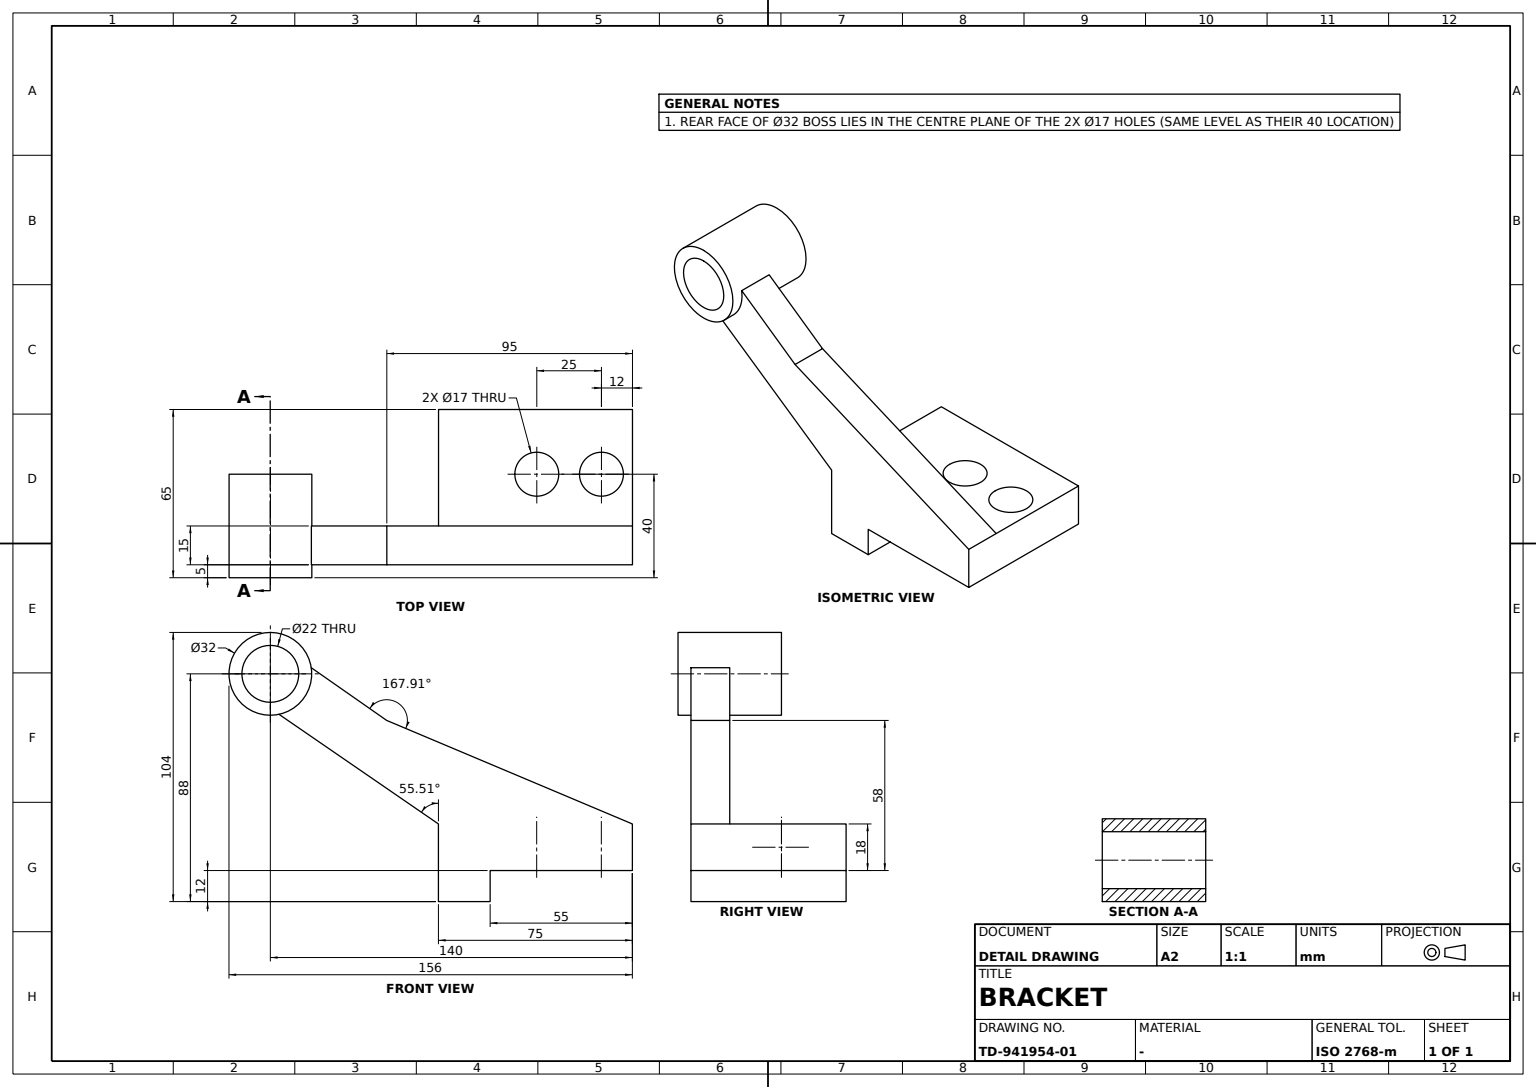
ISO-10303-21;
HEADER;
FILE_DESCRIPTION((''),'2;1');
FILE_NAME('','',(''),(''),'','','');
FILE_SCHEMA(('AUTOMOTIVE_DESIGN'));
ENDSEC;
DATA;
#1=APPLICATION_CONTEXT('');
#2=PRODUCT_CONTEXT('',#1,'mechanical');
#3=PRODUCT('','','',(#2));
#4=PRODUCT_DEFINITION_FORMATION('','',#3);
#5=PRODUCT_DEFINITION_CONTEXT('',#1,'design');
#6=PRODUCT_DEFINITION('','',#4,#5);
#7=PRODUCT_DEFINITION_SHAPE('','',#6);
#8=(LENGTH_UNIT()NAMED_UNIT(*)SI_UNIT(.MILLI.,.METRE.));
#9=(NAMED_UNIT(*)PLANE_ANGLE_UNIT()SI_UNIT($,.RADIAN.));
#10=(NAMED_UNIT(*)SI_UNIT($,.STERADIAN.)SOLID_ANGLE_UNIT());
#11=UNCERTAINTY_MEASURE_WITH_UNIT(LENGTH_MEASURE(0.005),#8,'distance_accuracy_value','');
#12=(GEOMETRIC_REPRESENTATION_CONTEXT(3)GLOBAL_UNCERTAINTY_ASSIGNED_CONTEXT((#11))GLOBAL_UNIT_ASSIGNED_CONTEXT((#8,#9,#10))REPRESENTATION_CONTEXT('',''));
#13=CARTESIAN_POINT('',(-140.,35.,92.));
#14=VERTEX_POINT('',#13);
#15=CARTESIAN_POINT('',(-140.,35.,76.));
#16=DIRECTION('',(0.,1.,0.));
#17=DIRECTION('',(0.,0.,1.));
#18=AXIS2_PLACEMENT_3D('',#15,#16,#17);
#19=CIRCLE('',#18,16.);
#20=EDGE_CURVE('',#14,#14,#19,.T.);
#21=ORIENTED_EDGE('',*,*,#20,.T.);
#22=EDGE_LOOP('',(#21));
#23=FACE_BOUND('',#22,.T.);
#24=CARTESIAN_POINT('',(-140.,35.,87.));
#25=VERTEX_POINT('',#24);
#26=CIRCLE('',#18,11.);
#27=EDGE_CURVE('',#25,#25,#26,.T.);
#28=ORIENTED_EDGE('',*,*,#27,.F.);
#29=EDGE_LOOP('',(#28));
#30=FACE_BOUND('',#29,.T.);
#31=CARTESIAN_POINT('',(0.,35.,0.));
#32=DIRECTION('',(-1.,0.,0.));
#33=AXIS2_PLACEMENT_3D('',#31,#16,#32);
#34=PLANE('',#33);
#35=ADVANCED_FACE('',(#23,#30),#34,.T.);
#36=CARTESIAN_POINT('',(-3.5,35.,0.));
#37=VERTEX_POINT('',#36);
#38=CARTESIAN_POINT('',(-12.,35.,0.));
#39=DIRECTION('',(1.,0.,0.));
#40=AXIS2_PLACEMENT_3D('',#38,#17,#39);
#41=CIRCLE('',#40,8.5);
#42=EDGE_CURVE('',#37,#37,#41,.T.);
#43=ORIENTED_EDGE('',*,*,#42,.F.);
#44=EDGE_LOOP('',(#43));
#45=FACE_BOUND('',#44,.T.);
#46=CARTESIAN_POINT('',(-20.5,35.,18.));
#47=VERTEX_POINT('',#46);
#48=CARTESIAN_POINT('',(-12.,35.,18.));
#49=DIRECTION('',(0.,0.,-1.));
#50=AXIS2_PLACEMENT_3D('',#48,#49,#32);
#51=CIRCLE('',#50,8.5);
#52=EDGE_CURVE('',#47,#47,#51,.T.);
#53=ORIENTED_EDGE('',*,*,#52,.F.);
#54=EDGE_LOOP('',(#53));
#55=FACE_BOUND('',#54,.T.);
#56=CARTESIAN_POINT('',(-12.,35.,10.));
#57=AXIS2_PLACEMENT_3D('',#56,#17,#39);
#58=CYLINDRICAL_SURFACE('',#57,8.5);
#59=ADVANCED_FACE('',(#45,#55),#58,.F.);
#60=CARTESIAN_POINT('',(-124.176279,0.,78.368516));
#61=VERTEX_POINT('',#60);
#62=CARTESIAN_POINT('',(-136.651894,0.,60.354228));
#63=VERTEX_POINT('',#62);
#64=CARTESIAN_POINT('',(-140.,0.,76.));
#65=AXIS2_PLACEMENT_3D('',#64,#16,#17);
#66=CIRCLE('',#65,16.);
#67=EDGE_CURVE('',#61,#63,#66,.T.);
#68=ORIENTED_EDGE('',*,*,#67,.T.);
#69=CARTESIAN_POINT('',(-75.,0.,18.));
#70=VERTEX_POINT('',#69);
#71=CARTESIAN_POINT('',(-15.646411,0.,-22.775315));
#72=DIRECTION('',(-0.824238161,0.,0.566243282));
#73=VECTOR('',#72,1000.);
#74=LINE('',#71,#73);
#75=EDGE_CURVE('',#70,#63,#74,.T.);
#76=ORIENTED_EDGE('',*,*,#75,.F.);
#77=CARTESIAN_POINT('',(-75.,0.,-12.));
#78=VERTEX_POINT('',#77);
#79=CARTESIAN_POINT('',(-75.,0.,0.));
#80=VECTOR('',#49,1000.);
#81=LINE('',#79,#80);
#82=EDGE_CURVE('',#70,#78,#81,.T.);
#83=ORIENTED_EDGE('',*,*,#82,.T.);
#84=CARTESIAN_POINT('',(-55.,0.,-12.));
#85=VERTEX_POINT('',#84);
#86=CARTESIAN_POINT('',(0.,0.,-12.));
#87=VECTOR('',#39,1000.);
#88=LINE('',#86,#87);
#89=EDGE_CURVE('',#78,#85,#88,.T.);
#90=ORIENTED_EDGE('',*,*,#89,.T.);
#91=CARTESIAN_POINT('',(-55.,0.,0.));
#92=VERTEX_POINT('',#91);
#93=VECTOR('',#17,1000.);
#94=LINE('',#91,#93);
#95=EDGE_CURVE('',#85,#92,#94,.T.);
#96=ORIENTED_EDGE('',*,*,#95,.T.);
#97=CARTESIAN_POINT('',(0.,0.,0.));
#98=VERTEX_POINT('',#97);
#99=LINE('',#97,#87);
#100=EDGE_CURVE('',#92,#98,#99,.T.);
#101=ORIENTED_EDGE('',*,*,#100,.T.);
#102=CARTESIAN_POINT('',(0.,0.,18.));
#103=VERTEX_POINT('',#102);
#104=LINE('',#97,#93);
#105=EDGE_CURVE('',#98,#103,#104,.T.);
#106=ORIENTED_EDGE('',*,*,#105,.T.);
#107=CARTESIAN_POINT('',(-95.,0.,58.));
#108=VERTEX_POINT('',#107);
#109=CARTESIAN_POINT('',(6.437647,0.,15.289412));
#110=DIRECTION('',(-0.921635375,0.,0.388057));
#111=VECTOR('',#110,1000.);
#112=LINE('',#109,#111);
#113=EDGE_CURVE('',#103,#108,#112,.T.);
#114=ORIENTED_EDGE('',*,*,#113,.T.);
#115=CARTESIAN_POINT('',(-3.905728,0.,-5.594645));
#116=DIRECTION('',(-0.819955841,0.,0.572426781));
#117=VECTOR('',#116,1000.);
#118=LINE('',#115,#117);
#119=EDGE_CURVE('',#108,#61,#118,.T.);
#120=ORIENTED_EDGE('',*,*,#119,.T.);
#121=EDGE_LOOP('',(#68,#76,#83,#90,#96,#101,#106,#114,#120));
#122=FACE_BOUND('',#121,.T.);
#123=AXIS2_PLACEMENT_3D('',#97,#16,#32);
#124=PLANE('',#123);
#125=ADVANCED_FACE('',(#122),#124,.F.);
#126=CARTESIAN_POINT('',(-140.,-5.,87.));
#127=VERTEX_POINT('',#126);
#128=CARTESIAN_POINT('',(-140.,-5.,76.));
#129=AXIS2_PLACEMENT_3D('',#128,#16,#17);
#130=CIRCLE('',#129,11.);
#131=EDGE_CURVE('',#127,#127,#130,.T.);
#132=ORIENTED_EDGE('',*,*,#131,.F.);
#133=EDGE_LOOP('',(#132));
#134=FACE_BOUND('',#133,.T.);
#135=ORIENTED_EDGE('',*,*,#27,.T.);
#136=EDGE_LOOP('',(#135));
#137=FACE_BOUND('',#136,.T.);
#138=CARTESIAN_POINT('',(-140.,-2.5,76.));
#139=AXIS2_PLACEMENT_3D('',#138,#16,#32);
#140=CYLINDRICAL_SURFACE('',#139,11.);
#141=ADVANCED_FACE('',(#134,#137),#140,.F.);
#142=ORIENTED_EDGE('',*,*,#75,.T.);
#143=CARTESIAN_POINT('',(-136.651894,15.,60.354228));
#144=VERTEX_POINT('',#143);
#145=VECTOR('',#16,1000.);
#146=LINE('',#62,#145);
#147=EDGE_CURVE('',#63,#144,#146,.T.);
#148=ORIENTED_EDGE('',*,*,#147,.T.);
#149=CARTESIAN_POINT('',(-75.,15.,18.));
#150=VERTEX_POINT('',#149);
#151=CARTESIAN_POINT('',(-15.646411,15.,-22.775315));
#152=LINE('',#151,#73);
#153=EDGE_CURVE('',#150,#144,#152,.T.);
#154=ORIENTED_EDGE('',*,*,#153,.F.);
#155=LINE('',#69,#145);
#156=EDGE_CURVE('',#70,#150,#155,.T.);
#157=ORIENTED_EDGE('',*,*,#156,.F.);
#158=EDGE_LOOP('',(#142,#148,#154,#157));
#159=FACE_BOUND('',#158,.T.);
#160=DIRECTION('',(-0.566243282,0.,-0.824238161));
#161=AXIS2_PLACEMENT_3D('',#69,#160,#72);
#162=PLANE('',#161);
#163=ADVANCED_FACE('',(#159),#162,.T.);
#164=CARTESIAN_POINT('',(-140.,-5.,92.));
#165=VERTEX_POINT('',#164);
#166=CIRCLE('',#129,16.);
#167=EDGE_CURVE('',#165,#165,#166,.T.);
#168=ORIENTED_EDGE('',*,*,#167,.T.);
#169=EDGE_LOOP('',(#168));
#170=FACE_BOUND('',#169,.T.);
#171=ORIENTED_EDGE('',*,*,#20,.F.);
#172=EDGE_LOOP('',(#171));
#173=FACE_BOUND('',#172,.T.);
#174=CARTESIAN_POINT('',(-124.176279,15.,78.368516));
#175=VERTEX_POINT('',#174);
#176=LINE('',#60,#145);
#177=EDGE_CURVE('',#61,#175,#176,.T.);
#178=ORIENTED_EDGE('',*,*,#177,.T.);
#179=CARTESIAN_POINT('',(-140.,15.,76.));
#180=AXIS2_PLACEMENT_3D('',#179,#16,#17);
#181=CIRCLE('',#180,16.);
#182=EDGE_CURVE('',#175,#144,#181,.T.);
#183=ORIENTED_EDGE('',*,*,#182,.T.);
#184=ORIENTED_EDGE('',*,*,#147,.F.);
#185=ORIENTED_EDGE('',*,*,#67,.F.);
#186=EDGE_LOOP('',(#178,#183,#184,#185));
#187=FACE_BOUND('',#186,.T.);
#188=CARTESIAN_POINT('',(-140.,7.5,76.));
#189=AXIS2_PLACEMENT_3D('',#188,#16,#32);
#190=CYLINDRICAL_SURFACE('',#189,16.);
#191=ADVANCED_FACE('',(#170,#173,#187),#190,.T.);
#192=CARTESIAN_POINT('',(-55.,60.,-12.));
#193=VERTEX_POINT('',#192);
#194=LINE('',#84,#145);
#195=EDGE_CURVE('',#85,#193,#194,.T.);
#196=ORIENTED_EDGE('',*,*,#195,.F.);
#197=ORIENTED_EDGE('',*,*,#89,.F.);
#198=CARTESIAN_POINT('',(-75.,60.,-12.));
#199=VERTEX_POINT('',#198);
#200=LINE('',#77,#145);
#201=EDGE_CURVE('',#78,#199,#200,.T.);
#202=ORIENTED_EDGE('',*,*,#201,.T.);
#203=CARTESIAN_POINT('',(0.,60.,-12.));
#204=LINE('',#203,#87);
#205=EDGE_CURVE('',#199,#193,#204,.T.);
#206=ORIENTED_EDGE('',*,*,#205,.T.);
#207=EDGE_LOOP('',(#196,#197,#202,#206));
#208=FACE_BOUND('',#207,.T.);
#209=AXIS2_PLACEMENT_3D('',#77,#17,#39);
#210=PLANE('',#209);
#211=ADVANCED_FACE('',(#208),#210,.F.);
#212=CARTESIAN_POINT('',(0.,15.,18.));
#213=VERTEX_POINT('',#212);
#214=LINE('',#102,#145);
#215=EDGE_CURVE('',#103,#213,#214,.T.);
#216=ORIENTED_EDGE('',*,*,#215,.T.);
#217=CARTESIAN_POINT('',(-95.,15.,58.));
#218=VERTEX_POINT('',#217);
#219=CARTESIAN_POINT('',(6.437647,15.,15.289412));
#220=LINE('',#219,#111);
#221=EDGE_CURVE('',#213,#218,#220,.T.);
#222=ORIENTED_EDGE('',*,*,#221,.T.);
#223=LINE('',#107,#145);
#224=EDGE_CURVE('',#108,#218,#223,.T.);
#225=ORIENTED_EDGE('',*,*,#224,.F.);
#226=ORIENTED_EDGE('',*,*,#113,.F.);
#227=EDGE_LOOP('',(#216,#222,#225,#226));
#228=FACE_BOUND('',#227,.T.);
#229=DIRECTION('',(-0.388057,0.,-0.921635375));
#230=AXIS2_PLACEMENT_3D('',#102,#229,#110);
#231=PLANE('',#230);
#232=ADVANCED_FACE('',(#228),#231,.F.);
#233=ORIENTED_EDGE('',*,*,#153,.T.);
#234=ORIENTED_EDGE('',*,*,#182,.F.);
#235=CARTESIAN_POINT('',(-3.905728,15.,-5.594645));
#236=LINE('',#235,#117);
#237=EDGE_CURVE('',#218,#175,#236,.T.);
#238=ORIENTED_EDGE('',*,*,#237,.F.);
#239=ORIENTED_EDGE('',*,*,#221,.F.);
#240=LINE('',#212,#87);
#241=EDGE_CURVE('',#150,#213,#240,.T.);
#242=ORIENTED_EDGE('',*,*,#241,.F.);
#243=EDGE_LOOP('',(#233,#234,#238,#239,#242));
#244=FACE_BOUND('',#243,.T.);
#245=CARTESIAN_POINT('',(0.,15.,0.));
#246=AXIS2_PLACEMENT_3D('',#245,#16,#32);
#247=PLANE('',#246);
#248=ADVANCED_FACE('',(#244),#247,.T.);
#249=ORIENTED_EDGE('',*,*,#131,.T.);
#250=EDGE_LOOP('',(#249));
#251=FACE_BOUND('',#250,.T.);
#252=ORIENTED_EDGE('',*,*,#167,.F.);
#253=EDGE_LOOP('',(#252));
#254=FACE_BOUND('',#253,.T.);
#255=CARTESIAN_POINT('',(0.,-5.,0.));
#256=AXIS2_PLACEMENT_3D('',#255,#16,#32);
#257=PLANE('',#256);
#258=ADVANCED_FACE('',(#251,#254),#257,.F.);
#259=ORIENTED_EDGE('',*,*,#156,.T.);
#260=CARTESIAN_POINT('',(-75.,60.,18.));
#261=VERTEX_POINT('',#260);
#262=EDGE_CURVE('',#150,#261,#155,.T.);
#263=ORIENTED_EDGE('',*,*,#262,.T.);
#264=CARTESIAN_POINT('',(-75.,60.,0.));
#265=LINE('',#264,#80);
#266=EDGE_CURVE('',#261,#199,#265,.T.);
#267=ORIENTED_EDGE('',*,*,#266,.T.);
#268=ORIENTED_EDGE('',*,*,#201,.F.);
#269=ORIENTED_EDGE('',*,*,#82,.F.);
#270=EDGE_LOOP('',(#259,#263,#267,#268,#269));
#271=FACE_BOUND('',#270,.T.);
#272=AXIS2_PLACEMENT_3D('',#69,#39,#49);
#273=PLANE('',#272);
#274=ADVANCED_FACE('',(#271),#273,.F.);
#275=CARTESIAN_POINT('',(-45.5,35.,18.));
#276=VERTEX_POINT('',#275);
#277=CARTESIAN_POINT('',(-37.,35.,18.));
#278=AXIS2_PLACEMENT_3D('',#277,#49,#32);
#279=CIRCLE('',#278,8.5);
#280=EDGE_CURVE('',#276,#276,#279,.T.);
#281=ORIENTED_EDGE('',*,*,#280,.T.);
#282=EDGE_LOOP('',(#281));
#283=FACE_BOUND('',#282,.T.);
#284=ORIENTED_EDGE('',*,*,#52,.T.);
#285=EDGE_LOOP('',(#284));
#286=FACE_BOUND('',#285,.T.);
#287=ORIENTED_EDGE('',*,*,#241,.T.);
#288=CARTESIAN_POINT('',(0.,60.,18.));
#289=VERTEX_POINT('',#288);
#290=EDGE_CURVE('',#213,#289,#214,.T.);
#291=ORIENTED_EDGE('',*,*,#290,.T.);
#292=VECTOR('',#32,1000.);
#293=LINE('',#288,#292);
#294=EDGE_CURVE('',#289,#261,#293,.T.);
#295=ORIENTED_EDGE('',*,*,#294,.T.);
#296=ORIENTED_EDGE('',*,*,#262,.F.);
#297=EDGE_LOOP('',(#287,#291,#295,#296));
#298=FACE_BOUND('',#297,.T.);
#299=AXIS2_PLACEMENT_3D('',#102,#49,#32);
#300=PLANE('',#299);
#301=ADVANCED_FACE('',(#283,#286,#298),#300,.F.);
#302=CARTESIAN_POINT('',(-28.5,35.,0.));
#303=VERTEX_POINT('',#302);
#304=CARTESIAN_POINT('',(-37.,35.,0.));
#305=AXIS2_PLACEMENT_3D('',#304,#17,#39);
#306=CIRCLE('',#305,8.5);
#307=EDGE_CURVE('',#303,#303,#306,.T.);
#308=ORIENTED_EDGE('',*,*,#307,.F.);
#309=EDGE_LOOP('',(#308));
#310=FACE_BOUND('',#309,.T.);
#311=ORIENTED_EDGE('',*,*,#280,.F.);
#312=EDGE_LOOP('',(#311));
#313=FACE_BOUND('',#312,.T.);
#314=CARTESIAN_POINT('',(-37.,35.,10.));
#315=AXIS2_PLACEMENT_3D('',#314,#17,#39);
#316=CYLINDRICAL_SURFACE('',#315,8.5);
#317=ADVANCED_FACE('',(#310,#313),#316,.F.);
#318=CARTESIAN_POINT('',(-55.,60.,0.));
#319=VERTEX_POINT('',#318);
#320=LINE('',#318,#93);
#321=EDGE_CURVE('',#193,#319,#320,.T.);
#322=ORIENTED_EDGE('',*,*,#321,.F.);
#323=ORIENTED_EDGE('',*,*,#205,.F.);
#324=ORIENTED_EDGE('',*,*,#266,.F.);
#325=ORIENTED_EDGE('',*,*,#294,.F.);
#326=CARTESIAN_POINT('',(0.,60.,0.));
#327=VERTEX_POINT('',#326);
#328=LINE('',#326,#93);
#329=EDGE_CURVE('',#327,#289,#328,.T.);
#330=ORIENTED_EDGE('',*,*,#329,.F.);
#331=LINE('',#326,#87);
#332=EDGE_CURVE('',#319,#327,#331,.T.);
#333=ORIENTED_EDGE('',*,*,#332,.F.);
#334=EDGE_LOOP('',(#322,#323,#324,#325,#330,#333));
#335=FACE_BOUND('',#334,.T.);
#336=AXIS2_PLACEMENT_3D('',#326,#16,#32);
#337=PLANE('',#336);
#338=ADVANCED_FACE('',(#335),#337,.T.);
#339=ORIENTED_EDGE('',*,*,#42,.T.);
#340=EDGE_LOOP('',(#339));
#341=FACE_BOUND('',#340,.T.);
#342=LINE('',#91,#145);
#343=EDGE_CURVE('',#92,#319,#342,.T.);
#344=ORIENTED_EDGE('',*,*,#343,.T.);
#345=ORIENTED_EDGE('',*,*,#332,.T.);
#346=LINE('',#97,#145);
#347=EDGE_CURVE('',#98,#327,#346,.T.);
#348=ORIENTED_EDGE('',*,*,#347,.F.);
#349=ORIENTED_EDGE('',*,*,#100,.F.);
#350=EDGE_LOOP('',(#344,#345,#348,#349));
#351=FACE_BOUND('',#350,.T.);
#352=ORIENTED_EDGE('',*,*,#307,.T.);
#353=EDGE_LOOP('',(#352));
#354=FACE_BOUND('',#353,.T.);
#355=AXIS2_PLACEMENT_3D('',#91,#17,#39);
#356=PLANE('',#355);
#357=ADVANCED_FACE('',(#341,#351,#354),#356,.F.);
#358=ORIENTED_EDGE('',*,*,#290,.F.);
#359=ORIENTED_EDGE('',*,*,#215,.F.);
#360=ORIENTED_EDGE('',*,*,#105,.F.);
#361=ORIENTED_EDGE('',*,*,#347,.T.);
#362=ORIENTED_EDGE('',*,*,#329,.T.);
#363=EDGE_LOOP('',(#358,#359,#360,#361,#362));
#364=FACE_BOUND('',#363,.T.);
#365=AXIS2_PLACEMENT_3D('',#97,#32,#17);
#366=PLANE('',#365);
#367=ADVANCED_FACE('',(#364),#366,.F.);
#368=ORIENTED_EDGE('',*,*,#95,.F.);
#369=ORIENTED_EDGE('',*,*,#195,.T.);
#370=ORIENTED_EDGE('',*,*,#321,.T.);
#371=ORIENTED_EDGE('',*,*,#343,.F.);
#372=EDGE_LOOP('',(#368,#369,#370,#371));
#373=FACE_BOUND('',#372,.T.);
#374=AXIS2_PLACEMENT_3D('',#84,#32,#17);
#375=PLANE('',#374);
#376=ADVANCED_FACE('',(#373),#375,.F.);
#377=ORIENTED_EDGE('',*,*,#119,.F.);
#378=ORIENTED_EDGE('',*,*,#224,.T.);
#379=ORIENTED_EDGE('',*,*,#237,.T.);
#380=ORIENTED_EDGE('',*,*,#177,.F.);
#381=EDGE_LOOP('',(#377,#378,#379,#380));
#382=FACE_BOUND('',#381,.T.);
#383=DIRECTION('',(-0.572426781,0.,-0.819955841));
#384=AXIS2_PLACEMENT_3D('',#107,#383,#116);
#385=PLANE('',#384);
#386=ADVANCED_FACE('',(#382),#385,.F.);
#387=CLOSED_SHELL('',(#35,#59,#125,#141,#163,#191,#211,#232,#248,#258,#274,#301,#317,#338,#357,#367,#376,#386));
#388=MANIFOLD_SOLID_BREP('',#387);
#389=ADVANCED_BREP_SHAPE_REPRESENTATION('',(#388),#12);
#390=SHAPE_DEFINITION_REPRESENTATION(#7,#389);
ENDSEC;
END-ISO-10303-21;
